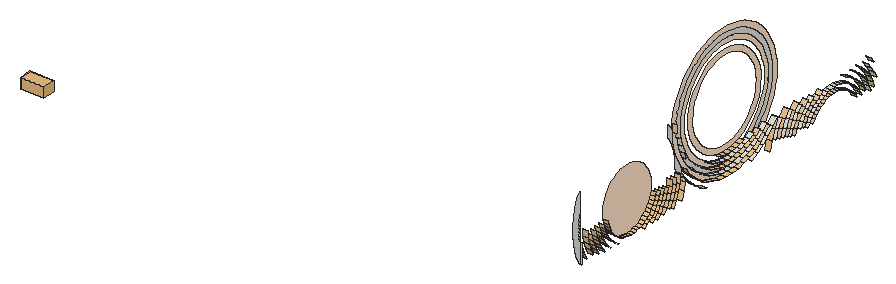
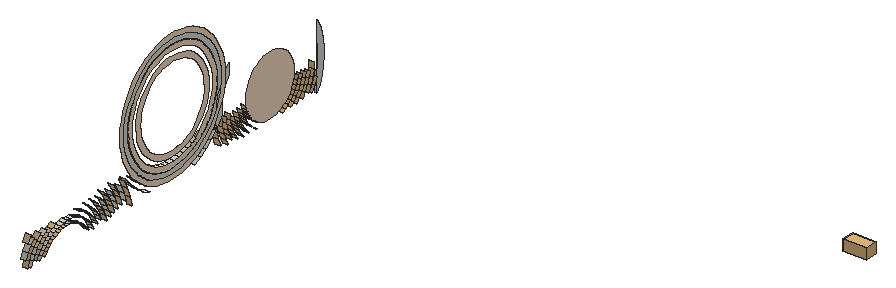
# SketchUp Ruby script. Lengths in inches.
U = 1.inch
M = Sketchup.active_model
def pt(a) = Geom::Point3d.new(a.map { |v| v * U })
def face(e, loops, mat)
  f = e.add_face(loops[0].map { |a| pt(a) })
  loops[1..].each { |l| e.add_face(l.map { |a| pt(a) }).erase! }
  f.material = f.back_material = mat if mat
  f
end
# faces: each face lists its corners as indices into pts; further lists are holes
def faces(e, pts, list, mat = nil) = list.each { |f| face(e, (f[0].is_a?(Array) ? f : [f]).map { |l| l.map { |i| pts[i] } }, mat) }
# xy, xz, yz: faces in a plane at the given z, y or x. An outline is a flat list of corners, or four numbers for a rectangle; further outlines are holes
def ring(l) = l.size == 4 ? [[l[0], l[1]], [l[2], l[1]], [l[2], l[3]], [l[0], l[3]]] : l.each_slice(2).to_a
def flat(e, list, mat, &to3) = list.each { |f| face(e, (f[0].is_a?(Array) ? f : [f]).map { |l| ring(l).map { |u, v| to3.(u, v) } }, mat) }
def xy(e, z, list, mat = nil) = flat(e, list, mat) { |x, y| [x, y, z] }
def xz(e, y, list, mat = nil) = flat(e, list, mat) { |x, z| [x, y, z] }
def yz(e, x, list, mat = nil) = flat(e, list, mat) { |y, z| [x, y, z] }
def lines(e, pts, list) = list.each { |a, b| e.add_line(pt(pts[a]), pt(pts[b])) }
# prism: a flat outline (further loops are holes) pulled along v
def prism(e, loops, v, mat = nil)
  f = face(e, loops, mat); d = Geom::Vector3d.new(v.map { |x| x * U })
  f.pushpull(f.normal.samedirection?(d) ? d.length : -d.length)
end
def box(e, o, s, mat = nil) = prism(e, [[o, [o[0] + s[0], o[1], o[2]], [o[0] + s[0], o[1] + s[1], o[2]], [o[0], o[1] + s[1], o[2]]]], [0, 0, s[2]], mat)
def at(x, y, z, deg = 0) = Geom::Transformation.translation(pt([x, y, z])) * Geom::Transformation.rotation(ORIGIN, Z_AXIS, deg.degrees)
def axes(o, x, y, z) = Geom::Transformation.new([*x, 0, *y, 0, *z, 0, *pt(o).to_a, 1])
def part(name) = M.definitions.add(name)
# library, detail: a bought-in or finely detailed component or shape, given as its bounding box
def library(name, o, s) = part(name).tap { |d| box(d.entities, o, s) }
def detail(e, o, s) = box(e.add_group.entities, o, s)
def put(e, d, t, mat = nil) = e.add_instance(d, t).tap { |i| i.material = mat if mat }
def group(e, t, mat = nil) = e.add_group.tap { |g| g.transformation = t; g.material = mat if mat }.entities
root = M.entities
M.materials.add("[Color C02]").color = [255, 228, 201]
M.materials.add("images").color = [235, 194, 141]
c1 = library("Group\#240",[-0.66,-0.65,0],[9.25,4.94,4.13])
xy(root,39.7,[[183.82,116.84,185.82,119.625]])
xy(root,41.7,[[183.82,116.96,185.82,119.51]],"images")
xz(root,46.5625,[[183.82,37.01,184.63,44.88]])
yz(root,183.82,[[46.5625,37.01,45.42,39.3125,44.37,42.24,43.67,45.27,43.32,48.36,43.34,51.47,43.71,54.56,44.44,57.58,45.52,60.49,46.5625,62.54,46.5625,54.71,46.41,54.07,46.07,51.3,46.05,48.51,46.36,45.73,46.5625,44.88],[[116.84,39.7,119.625,39.7,122.39,40.02,125.1,40.66,127.72,41.6,130.21,42.85,132.53,44.375,134.67,46.16,136.58,48.18,138.25,50.41,139.64,52.82,140.75,55.375,141.55,58.04,142.04,60.78,142.2,63.56,142.05,66.34,141.57,69.08,140.77,71.75,139.68,74.3,138.29,76.72,136.63,78.95,134.72,80.98,132.59,82.77,130.27,84.3,127.78,85.56,125.17,86.51,122.46,87.16,119.7,87.49,116.91,87.49,114.15,87.17,111.44,86.53,108.82,85.59,106.33,84.34,104.01,82.8125,101.87,81.03,99.96,79.01,98.29,76.78,96.9,74.37,95.79,71.8125,94.99,69.15,94.5,66.41,94.34,63.63,94.49,60.85,94.59,60.33,94.625,60.25,95.67,57.32,96.375,54.3,96.42,53.93,96.87,52.88,98.25,50.47,99.91,48.24,101.82,46.21,103.95,44.42,106.27,42.88,108.76,41.63,111.37,40.68,114.08,40.03],[116.96,41.7,114.43,42,111.95,42.59,109.55,43.47,107.27,44.62,105.15,46.02,103.19,47.66,101.45,49.52,99.93,51.57,98.65,53.78,97.65,56.125,96.92,58.57,96.48,61.08,96.34,63.63,96.49,66.17,96.94,68.68,97.67,71.13,98.68,73.47,99.96,75.67,101.49,77.72,103.24,79.57,105.2,81.21,107.33,82.61,109.61,83.75,112.01,84.62,114.49,85.2,117.03,85.49,119.58,85.49,122.11,85.19,124.59,84.6,126.99,83.72,129.27,82.57,131.4,81.17,133.35,79.53,135.09,77.67,136.61,75.62,137.89,73.41,138.89,71.07,139.62,68.62,140.06,66.11,140.2,63.5625,140.05,61.02,139.61,58.5,138.87,56.0625,137.86,53.72,136.58,51.51,135.05,49.47,133.3,47.62,131.34,45.98,129.21,44.58,126.93,43.44,124.53,42.57,122.05,41.99,119.51,41.7]],[[116.96,41.7,119.51,41.7,122.05,41.99,124.53,42.57,126.93,43.44,129.21,44.58,131.34,45.98,133.3,47.62,135.05,49.47,136.58,51.51,137.86,53.72,138.87,56.0625,139.61,58.5,140.05,61.02,140.2,63.5625,140.06,66.11,139.62,68.62,138.89,71.07,137.89,73.41,136.61,75.62,135.09,77.67,133.35,79.53,131.4,81.17,129.27,82.57,126.99,83.72,124.59,84.6,122.11,85.19,119.58,85.49,117.03,85.49,114.49,85.2,112.01,84.62,109.61,83.75,107.33,82.61,105.2,81.21,103.24,79.57,101.49,77.72,99.96,75.67,98.68,73.47,97.67,71.13,96.94,68.68,96.49,66.17,96.34,63.63,96.48,61.08,96.92,58.57,97.65,56.125,98.65,53.78,99.93,51.57,101.45,49.52,103.19,47.66,105.15,46.02,107.27,44.62,109.55,43.47,111.95,42.59,114.43,42],[116.96,41.71,114.43,42.01,111.95,42.6,109.56,43.48,107.28,44.625,105.15,46.03,103.2,47.67,101.45,49.53,99.94,51.57,98.66,53.78,97.66,56.125,96.93,58.57,96.49,61.08,96.35,63.63,96.5,66.17,96.94,68.68,97.68,71.125,98.69,73.46,99.97,75.67,101.5,77.71,103.25,79.5625,105.2,81.2,107.34,82.6,109.62,83.74,112.01,84.61,114.5,85.19,117.03,85.48,119.58,85.48,122.11,85.18,124.59,84.59,126.98,83.71,129.26,82.56,131.39,81.16,133.34,79.52,135.09,77.66,136.61,75.61,137.88,73.4,138.88,71.0625,139.61,68.62,140.05,66.11,140.19,63.5625,140.04,61.02,139.6,58.51,138.86,56.07,137.85,53.73,136.57,51.52,135.04,49.48,133.29,47.625,131.34,45.99,129.2,44.59,126.92,43.45,124.53,42.58,122.05,42,119.51,41.71]],[46.5625,44.88,46.36,45.73,46.05,48.51,46.07,51.3,46.41,54.07,46.5625,54.71],[96.47,46.17,96.71,48.1,96.71,49.2,96.58,49.375,95.08,51.99,93.89,54.76,93.03,57.65,92.51,60.62,92.34,63.63,92.38,64.36,91.55,65.64,90.53,66.87,90.34,63.64,90.41,62.38,90.86,61.68,92.1,59.18,93.05,56.55,93.68,53.83,93.99,51.06,93.98,49.89,94.91,48.28],
  [96.42,53.93,96.375,54.3,95.67,57.32,94.625,60.25,94.59,60.33,94.97,58.11,95.77,55.44]])
yz(root,183.82,[[[119.74,37.7,122.74,38.05,125.67,38.74,128.51,39.77,131.2,41.12,133.73,42.77,136.04,44.7,138.11,46.89,139.92,49.3125,141.43,51.92,142.63,54.6875,143.5,57.58,144.02,60.55,144.2,63.56,144.03,66.57,143.51,69.54,142.65,72.43,141.46,75.2,139.96,77.8125,138.16,80.23,136.1,82.43,133.79,84.375,131.27,86.03,128.58,87.39,125.75,88.43,122.8125,89.13,119.82,89.48,116.8,89.49,113.81,89.14,110.87,88.45,108.03,87.42,105.34,86.07,102.81,84.42,100.5,82.49,98.43,80.29,96.625,77.88,95.11,75.27,93.91,72.5,93.04,69.61,92.52,66.64,92.38,64.36,92.34,63.63,92.51,60.62,93.03,57.65,93.89,54.76,95.08,51.99,96.58,49.375,96.71,49.2,98.38,46.95,100.45,44.76,102.75,42.82,105.27,41.15,107.96,39.8,110.8,38.76,113.73,38.0625,116.72,37.71],[116.84,39.7,114.08,40.03,111.37,40.68,108.76,41.63,106.27,42.88,103.95,44.42,101.82,46.21,99.91,48.24,98.25,50.47,96.87,52.88,96.42,53.93,95.77,55.44,94.97,58.11,94.59,60.33,94.49,60.85,94.34,63.63,94.5,66.41,94.99,69.15,95.79,71.8125,96.9,74.37,98.29,76.78,99.96,79.01,101.87,81.03,104.01,82.8125,106.33,84.34,108.82,85.59,111.44,86.53,114.15,87.17,116.91,87.49,119.7,87.49,122.46,87.16,125.17,86.51,127.78,85.56,130.27,84.3,132.59,82.77,134.72,80.98,136.63,78.95,138.29,76.72,139.68,74.3,140.77,71.75,141.57,69.08,142.05,66.34,142.2,63.56,142.04,60.78,141.55,58.04,140.75,55.375,139.64,52.82,138.25,50.41,136.58,48.18,134.67,46.16,132.53,44.375,130.21,42.85,127.72,41.6,125.1,40.66,122.39,40.02,119.625,39.7]],[69.96,37.78,71.35,37.86,72.73,38.09,74.07,38.49,75.35,39.03,76.57,39.72,77.6875,40.55,78.71,41.51,79.61,42.57,80.38,43.73,81.02,44.98,81.5,46.28,81.83,47.64,82,49.03,82,50.42,81.85,51.81,81.53,53.17,81.0625,54.48,80.44,55.73,79.68,56.9,78.79,57.97,77.78,58.9375,76.66,59.78,75.46,60.48,74.18,61.04,72.85,61.45,71.47,61.69,70.08,61.78,68.6875,61.71,67.3125,61.47,65.97,61.08,64.6875,60.53,63.48,59.84,62.35,59.01,61.33,58.0625,60.43,57,59.66,55.83,59.03,54.59,58.54,53.28,58.21,51.93,58.04,50.54,58.04,49.14,58.19,47.76,58.51,46.4,58.98,45.08,59.6,43.83,60.36,42.66,61.25,41.59,62.26,40.63,63.38,39.79,64.58,39.09,65.86,38.53,67.2,38.12,68.57,37.87],[[116.96,41.71,119.51,41.71,122.05,42,124.53,42.58,126.92,43.45,129.2,44.59,131.34,45.99,133.29,47.625,135.04,49.48,136.57,51.52,137.85,53.73,138.86,56.07,139.6,58.51,140.04,61.02,140.19,63.5625,140.05,66.11,139.61,68.62,138.88,71.0625,137.88,73.4,136.61,75.61,135.09,77.66,133.34,79.52,131.39,81.16,129.26,82.56,126.98,83.71,124.59,84.59,122.11,85.18,119.58,85.48,117.03,85.48,114.5,85.19,112.01,84.61,109.62,83.74,107.34,82.6,105.2,81.2,103.25,79.5625,101.5,77.71,99.97,75.67,98.69,73.46,97.68,71.125,96.94,68.68,96.5,66.17,96.35,63.63,96.49,61.08,96.93,58.57,97.66,56.125,98.66,53.78,99.94,51.57,101.45,49.53,103.2,47.67,105.15,46.03,107.28,44.625,109.56,43.48,111.95,42.6,114.43,42.01],[119.4,43.69,117.08,43.7,114.78,43.97,112.52,44.51,110.35,45.3,108.28,46.35,106.34,47.62,104.57,49.12,102.98,50.8,101.6,52.67,100.44,54.67,99.53,56.8,98.87,59.03,98.47,61.31,98.34,63.625,98.47,65.9375,98.88,68.22,99.55,70.44,100.47,72.57,101.63,74.57,103.02,76.43,104.61,78.11,106.39,79.6,108.33,80.87,110.4,81.91,112.58,82.7,114.84,83.23,117.14,83.5,119.46,83.49,121.76,83.22,124.02,82.68,126.19,81.89,128.26,80.84,130.2,79.57,131.97,78.07,133.56,76.39,134.94,74.52,136.1,72.51,137.01,70.38,137.67,68.16,138.07,65.88,138.2,63.56,138.07,61.25,137.66,58.97,136.99,56.75,136.07,54.62,134.91,52.62,133.52,50.76,131.93,49.07,130.15,47.59,128.21,46.32,126.14,45.28,123.96,44.49,121.7,43.96]],[[119.29,45.6875,121.36,45.93,123.39,46.41,125.35,47.12,127.21,48.05,128.96,49.19,130.56,50.53,131.99,52.05,133.24,53.72,134.29,55.52,135.11,57.44,135.72,59.43,136.08,61.49,136.2,63.57,136.09,65.65,135.73,67.7,135.13,69.7,134.31,71.62,133.27,73.43,132.03,75.1,130.6,76.62,129,77.96,127.26,79.11,125.4,80.05,123.44,80.77,121.41,81.25,119.34,81.5,117.25,81.5,115.18,81.26,113.15,80.78,111.19,80.07,109.33,79.14,107.58,78,105.98,76.66,104.55,75.14,103.3,73.47,102.26,71.67,101.43,69.75,100.83,67.76,100.46,65.7,100.34,63.62,100.45,61.54,100.8125,59.48,101.41,57.49,102.23,55.57,103.27,53.76,104.51,52.09,105.94,50.57,107.54,49.23,109.28,48.08,111.14,47.14,113.1,46.42,115.13,45.9375,117.2,45.69],[117.32,47.6875,115.48,47.91,113.68,48.34,111.9375,48.97,110.28,49.81,108.74,50.83,107.32,52.02,106.05,53.37,104.94,54.86,104.02,56.46,103.29,58.17,102.76,59.94,102.44,61.77,102.34,63.62,102.45,65.47,102.77,67.29,103.31,69.07,104.04,70.77,104.97,72.37,106.08,73.86,107.35,75.2,108.77,76.39,110.32,77.41,111.98,78.24,113.72,78.87,115.53,79.29,117.37,79.5,119.22,79.5,121.0625,79.28,122.86,78.85,124.6,78.22,126.26,77.38,127.81,76.36,129.22,75.17,130.49,73.82,131.6,72.33,132.52,70.72,133.25,69.02,133.78,67.25,134.1,65.42,134.2,63.57,134.09,61.72,133.77,59.9,133.24,58.12,132.5,56.42,131.57,54.82,130.46,53.33,129.1875,51.99,127.77,50.8,126.22,49.78,124.56,48.95,122.82,48.32,121.01,47.9,119.17,47.6875]]],"[Color C02]")
p = [[183.82,139.31,40.71],[183.82,138.46,37.03],[185.82,138.46,37.03],[185.82,139.31,40.71],[183.82,187.32,38.99],[183.82,188.07,36.98],
  [185.82,188.07,36.98],[185.82,187.32,38.99],[183.82,76.24,37.24],[183.82,77.66,38.05],[185.82,77.66,38.05],[185.82,76.24,37.24],
  [183.82,157.14,37.23],[183.82,157.89,38.73],[185.82,157.89,38.73],[185.82,157.14,37.23],[183.82,62.27,38.125],[183.82,63.68,37.3],
  [185.82,63.68,37.3],[185.82,62.27,38.125],[183.82,151.62,39.57],[183.82,150.82,37.34],[185.82,150.82,37.34],[185.82,151.62,39.57],
  [183.82,83.05,37.37],[183.82,84.41,38.96],[185.82,84.41,38.96],[185.82,83.05,37.37],[183.82,182.89,38.88],[183.82,183.66,37.39],
  [185.82,183.66,37.39],[185.82,182.89,38.88],[183.82,55.53,39.11],[183.82,56.87,37.5],[185.82,56.87,37.5],[185.82,55.53,39.11],
  [183.82,81.6,38.75],[183.82,80.24,37.48],[185.82,80.24,37.48],[185.82,81.6,38.75],[183.82,59.68,37.58],[183.82,58.33,38.86],
  [185.82,58.33,38.86],[185.82,59.68,37.58],[183.82,189.98,37.57],[183.82,189.15,39.79],[185.82,189.15,39.79],[185.82,189.98,37.57],
  [183.82,92.01,40.17],[183.82,90.75,37.68],[185.82,90.75,37.68],[185.82,92.01,40.17],[183.82,116.72,37.71],[183.82,113.73,38.0625],
  [185.82,113.73,38.0625],[185.82,116.72,37.71],[183.82,119.74,37.7],[185.82,119.74,37.7],[183.82,122.74,38.05],[185.82,122.74,38.05],
  [183.82,160.41,38.96],[183.82,159.625,37.74],[185.82,159.625,37.74],[185.82,160.41,38.96],[183.82,69.96,37.78],[183.82,68.57,37.87],
  [185.82,68.57,37.87],[185.82,69.96,37.78],[183.82,71.35,37.86],[185.82,71.35,37.86],[183.82,87.29,39.7],[183.82,86,37.76],
  [185.82,86,37.76],[185.82,87.29,39.7],[183.82,49.18,37.89],[183.82,47.9375,40.39],[184.63,47.9375,40.39],[184.63,49.18,37.89],
  [183.82,53.92,37.92],[183.82,52.65,39.87],[185.82,52.65,39.87],[185.82,53.92,37.92],[183.82,67.2,38.12],[185.82,67.2,38.12],
  [183.82,72.73,38.09],[185.82,72.73,38.09],[183.82,129.3,37.93],[183.82,132.2,39.38],[185.82,132.2,39.38],[185.82,129.3,37.93],
  [183.82,148.9,37.9],[183.82,149.78,40.35],[185.82,149.78,40.35],[185.82,148.9,37.9],[183.82,181.17,37.87],[183.82,180.37,39.08],
  [185.82,180.37,39.08],[185.82,181.17,37.87],[183.82,78.97,39.01],[185.82,78.97,39.01],[183.82,104.27,39.42],[183.82,107.17,37.96],
  [185.82,107.17,37.96],[185.82,104.27,39.42],[183.82,125.67,38.74],[185.82,125.67,38.74],[183.82,156.15,39.72],[183.82,155.3,38.01],
  [185.82,155.3,38.01],[185.82,156.15,39.72],[183.82,60.97,39.1],[185.82,60.97,39.1],[183.82,65.86,38.53],[185.82,65.86,38.53],
  [183.82,74.07,38.49],[185.82,74.07,38.49],[183.82,110.8,38.76],[185.82,110.8,38.76],[183.82,185.49,38.1875],[183.82,184.62,39.89],
  [185.82,184.62,39.89],[185.82,185.49,38.1875],[183.82,64.58,39.09],[185.82,64.58,39.09],[183.82,75.35,39.03],[185.82,75.35,39.03],
  [183.82,147.9375,41.14],[183.82,146.98,38.46],[185.82,146.98,38.46],[185.82,147.9375,41.14],[183.82,82.81,40.17],[185.82,82.81,40.17],
  [183.82,89.02,38.6875],[183.82,90.18,40.97],[185.82,90.18,40.97],[185.82,89.02,38.6875],[183.82,128.51,39.77],[185.82,128.51,39.77],
  [183.82,158.8,40.14],[185.82,158.8,40.14],[183.82,107.96,39.8],[185.82,107.96,39.8],[183.82,153.46,38.79],[183.82,154.41,40.71],
  [185.82,154.41,40.71],[185.82,153.46,38.79],[183.82,49.78,41.17],[183.82,50.91,38.88],[185.82,50.91,38.88],[185.82,49.78,41.17],
  [183.82,57.14,40.29],[185.82,57.14,40.29],[183.82,181.96,40.28],[185.82,181.96,40.28],[183.82,76.57,39.72],[185.82,76.57,39.72],
  [183.82,80.16,40.125],[185.82,80.16,40.125],[183.82,85.5625,40.71],[185.82,85.5625,40.71],[183.82,145.0625,39.02],[183.82,146.1,41.92],
  [185.82,146.1,41.92],[185.82,145.0625,39.02],[183.82,161.34,40.07],[185.82,161.34,40.07],[183.82,186.35,40.9],[185.82,186.35,40.9],
  [183.82,54.39,40.86],[185.82,54.39,40.86],[183.82,59.79,40.23],[185.82,59.79,40.23],[183.82,63.38,39.79],[185.82,63.38,39.79],
  [183.82,94.52,39.07],[183.82,95.6,41.99],[185.82,95.6,41.99],[185.82,94.52,39.07],[183.82,179.43,40.18],[185.82,179.43,40.18],
  [183.82,101.56,41.21],[185.82,101.56,41.21],[183.82,134.92,41.16],[185.82,134.92,41.16],[183.82,144.26,42.7],[183.82,143.14,39.58],
  [185.82,143.14,39.58],[185.82,144.26,42.7],[183.82,152.67,41.7],[185.82,152.67,41.7],[183.82,77.6875,40.55],[185.82,77.6875,40.55],
  [183.82,88.35,41.77],[185.82,88.35,41.77],[183.82,114.08,40.03],[183.82,116.84,39.7],[185.82,116.84,39.7],[185.82,114.08,40.03],
  [183.82,119.625,39.7],[183.82,122.39,40.02],[185.82,122.39,40.02],[185.82,119.625,39.7],[183.82,157.19,41.33],[185.82,157.19,41.33],
  [183.82,62.26,40.63],[185.82,62.26,40.63],[183.82,105.27,41.15],[185.82,105.27,41.15],[183.82,131.2,41.12],[185.82,131.2,41.12],
  [183.82,188.07,41.91],[185.82,188.07,41.91],[183.82,51.62,41.95],[185.82,51.62,41.95],[183.82,183.5625,41.48],[185.82,183.5625,41.48],
  [183.82,111.37,40.68],[185.82,111.37,40.68],[183.82,125.1,40.66],[185.82,125.1,40.66],[183.82,81.21,41.37],[185.82,81.21,41.37],
  [183.82,141.22,40.15],[183.82,142.42,43.48],[185.82,142.42,43.48],[185.82,141.22,40.15],[183.82,159.875,41.43],[185.82,159.875,41.43],
  [183.82,162.38,41.07],[185.82,162.38,41.07],[183.82,58.75,41.48],[185.82,58.75,41.48],[183.82,83.84,41.71],[185.82,83.84,41.71],
  [183.82,92.98,42.79],[185.82,92.98,42.79],[183.82,178.37,41.16],[185.82,178.37,41.16],[183.82,56.125,41.85],[185.82,56.125,41.85],
  [183.82,180.88,41.56],[185.82,180.88,41.56],[183.82,47,43.01],[184.63,47,43.01],[183.82,150.9375,42.69],[185.82,150.9375,42.69],
  [183.82,61.25,41.59],[185.82,61.25,41.59],[183.82,78.71,41.51],[185.82,78.71,41.51],[183.82,189.8,42.92],[183.82,190.98,40.6],
  [185.82,190.98,40.6],[185.82,189.8,42.92],[183.82,86.51,42.57],[185.82,86.51,42.57],[183.82,108.76,41.63],[185.82,108.76,41.63],
  [183.82,127.72,41.6],[185.82,127.72,41.6],[183.82,140.57,44.26],[185.82,140.57,44.26],[183.82,155.58,42.51],[185.82,155.58,42.51],
  [183.82,53.46,42.74],[185.82,53.46,42.74],[183.82,185.16,42.6875],[185.82,185.16,42.6875],[183.82,91.06,43.37],[185.82,91.06,43.37],
  [183.82,133.73,42.77],[185.82,133.73,42.77],[183.82,149.2,43.68],[185.82,149.2,43.68],[183.82,163.54,41.94],[185.82,163.54,41.94],
  [183.82,48.91,43.58],[185.82,48.91,43.58],[183.82,99.07,43.3],[185.82,99.07,43.3],[183.82,102.75,42.82],[185.82,102.75,42.82],
  [183.82,137.41,43.25],[185.82,137.41,43.25],[183.82,177.21,42.02],[185.82,177.21,42.02],[183.82,158.41,42.8],[185.82,158.41,42.8],
  [183.82,82.11,42.72],[185.82,82.11,42.72],[183.82,161.09,42.59],[185.82,161.09,42.59],[183.82,57.86,42.84],[185.82,57.86,42.84],
  [183.82,79.61,42.57],[185.82,79.61,42.57],[183.82,182.32,42.94],[185.82,182.32,42.94],[183.82,60.36,42.66],[185.82,60.36,42.66],
  [183.82,106.27,42.88],[185.82,106.27,42.88],[183.82,130.21,42.85],[185.82,130.21,42.85],[183.82,179.65,42.7],[185.82,179.65,42.7],
  [183.82,84.68,43.375],[185.82,84.68,43.375],[183.82,116.96,41.7],[183.82,114.43,42],[185.82,114.43,42],[185.82,116.96,41.7],
  [183.82,122.05,41.99],[183.82,119.51,41.7],[185.82,119.51,41.7],[185.82,122.05,41.99],[183.82,153.97,43.7],[185.82,153.97,43.7],
  [183.82,89.15,43.95],[185.82,89.15,43.95],[183.82,55.3,43.52],[185.82,55.3,43.52],[183.82,147.46,44.67],[185.82,147.46,44.67],
  [183.82,164.79,42.67],[185.82,164.79,42.67],[183.82,186.76,43.89],[185.82,186.76,43.89],[183.82,50.83,44.14],[185.82,50.83,44.14],
  [183.82,96.33,45.01],[185.82,96.33,45.01],[183.82,111.95,42.59],[185.82,111.95,42.59],[183.82,124.53,42.57],[185.82,124.53,42.57],
  [183.82,175.95,42.74],[185.82,175.95,42.74],[183.82,156.95,44.16],[185.82,156.95,44.16],[183.82,80.38,43.73],[185.82,80.38,43.73],
  [183.82,87.24,44.54],[185.82,87.24,44.54],[183.82,109.55,43.47],[185.82,109.55,43.47],[183.82,126.93,43.44],[185.82,126.93,43.44],
  [183.82,162.43,43.6],[185.82,162.43,43.6],[183.82,52.75,44.71],[185.82,52.75,44.71],[183.82,59.6,43.83],[185.82,59.6,43.83],
  [183.82,82.85,44.17],[185.82,82.85,44.17],[183.82,145.72,45.66],[185.82,145.72,45.66],[183.82,152.36,44.88],[185.82,152.36,44.88],
  [183.82,166.11,43.25],[185.82,166.11,43.25],[183.82,174.62,43.3],[185.82,174.62,43.3],[183.82,178.3,43.7],[185.82,178.3,43.7],
  [183.82,183.77,44.32],[185.82,183.77,44.32],[183.82,57.14,44.3],[185.82,57.14,44.3],[183.82,93.64,45.5],[185.82,93.64,45.5],
  [183.82,100.45,44.76],[185.82,100.45,44.76],[183.82,132.53,44.375],[185.82,132.53,44.375],[183.82,136.04,44.7],[185.82,136.04,44.7],
  [183.82,159.79,44.12],[185.82,159.79,44.12],[183.82,103.95,44.42],[185.82,103.95,44.42],[183.82,180.93,44.24],[185.82,180.93,44.24],
  [183.82,188.35,45.09],[185.82,188.35,45.09],[183.82,46.5625,44.88],[184.63,46.5625,44.88],[183.82,139.64,45.61],[185.82,139.64,45.61],
  [183.82,96.84,45.67],[185.82,96.84,45.67],[183.82,167.49,43.67],[185.82,167.49,43.67],[183.82,173.23,43.71],[185.82,173.23,43.71],
  [183.82,85.33,45.12],[185.82,85.33,45.12],[183.82,91.67,45.86],[185.82,91.67,45.86],[183.82,129.21,44.58],[185.82,129.21,44.58],
  [183.82,54.67,45.27],[185.82,54.67,45.27],[183.82,107.27,44.62],[185.82,107.27,44.62],[183.82,143.99,46.65],[185.82,143.99,46.65],
  [183.82,48.34,46.07],[185.82,48.34,46.07],[183.82,163.88,44.45],[185.82,163.88,44.45],[183.82,81.02,44.98],[185.82,81.02,44.98],
  [183.82,114.78,43.97],[183.82,117.08,43.7],[185.82,117.08,43.7],[185.82,114.78,43.97],[183.82,119.4,43.69],[185.82,119.4,43.69],
  [183.82,121.7,43.96],[185.82,121.7,43.96],[183.82,150.75,46.07],[185.82,150.75,46.07],[183.82,155.49,45.53],[185.82,155.49,45.53],
  [183.82,168.92,43.93],[185.82,168.92,43.93],[183.82,171.81,43.95],[185.82,171.81,43.95],[183.82,176.84,44.53],[185.82,176.84,44.53],
  [183.82,58.98,45.08],[185.82,58.98,45.08],[183.82,170.36,44.03],[185.82,170.36,44.03],[183.82,185.22,45.7],[185.82,185.22,45.7],
  [183.82,89.7,46.21],[185.82,89.7,46.21],[183.82,112.52,44.51],[185.82,112.52,44.51],[183.82,123.96,44.49],[185.82,123.96,44.49],
  [183.82,50.31,46.41],[185.82,50.31,46.41],[183.82,161.32,45.27],[185.82,161.32,45.27],[183.82,83.41,45.7],[185.82,83.41,45.7],
  [183.82,158.5,45.64],[185.82,158.5,45.64],[183.82,179.39,45.375],[185.82,179.39,45.375],[183.82,56.59,45.83],[185.82,56.59,45.83],
  [183.82,142.25,47.64],[185.82,142.25,47.64],[183.82,182.2,45.78],[185.82,182.2,45.78],[183.82,101.82,46.21],[185.82,101.82,46.21],
  [183.82,134.67,46.16],[185.82,134.67,46.16],[183.82,87.73,46.57],[185.82,87.73,46.57],[183.82,110.35,45.3],[185.82,110.35,45.3],
  [183.82,126.14,45.28],[185.82,126.14,45.28],[183.82,165.42,45.125],[185.82,165.42,45.125],[183.82,175.29,45.18],[185.82,175.29,45.18],
  [183.82,105.15,46.02],[185.82,105.15,46.02],[183.82,131.34,45.98],[185.82,131.34,45.98],[183.82,52.28,46.75],[185.82,52.28,46.75],
  [183.82,138.11,46.89],[185.82,138.11,46.89],[183.82,149.14,47.25],[185.82,149.14,47.25],[183.82,98.38,46.95],[185.82,98.38,46.95],
  [183.82,154.02,46.89],[185.82,154.02,46.89],[183.82,81.5,46.28],[185.82,81.5,46.28],[183.82,96.47,46.17],[185.82,96.47,46.17],
  [183.82,58.51,46.4],[185.82,58.51,46.4],[183.82,85.76,46.93],[185.82,85.76,46.93],[183.82,167.02,45.62],[185.82,167.02,45.62],
  [183.82,186.66,47.08],[185.82,186.66,47.08],[183.82,173.68,45.66],[185.82,173.68,45.66],[183.82,54.25,47.08],[185.82,54.25,47.08],
  [183.82,108.28,46.35],[185.82,108.28,46.35],[183.82,128.21,46.32],[185.82,128.21,46.32],[183.82,162.97,46.23],[185.82,162.97,46.23],
  [183.82,177.72,46.32],[185.82,177.72,46.32],[183.82,93.97,48.27],[185.82,93.97,48.27],[183.82,157.21,47.17],[185.82,157.21,47.17],
  [183.82,141.59,48.21],[185.82,141.59,48.21],[183.82,160.21,46.93],[185.82,160.21,46.93],[183.82,168.67,45.92],[185.82,168.67,45.92],
  [183.82,83.8,47.28],[185.82,83.8,47.28],[183.82,117.2,45.69],[183.82,115.13,45.9375],[185.82,115.13,45.9375],[185.82,117.2,45.69],
  [183.82,119.29,45.6875],[185.82,119.29,45.6875],[183.82,121.36,45.93],[185.82,121.36,45.93],[183.82,147.52,48.4375],[185.82,147.52,48.4375],
  [183.82,172.03,45.9375],[185.82,172.03,45.9375],[183.82,183.48,47.32],[185.82,183.48,47.32],[183.82,56.22,47.42],[185.82,56.22,47.42],
  [183.82,180.47,47.05],[185.82,180.47,47.05],[183.82,91.98,48.4],[185.82,91.98,48.4],[183.82,113.1,46.42],[185.82,113.1,46.42],
  [183.82,123.39,46.41],[185.82,123.39,46.41],[183.82,170.35,46.03],[185.82,170.35,46.03],[183.82,103.19,47.66],[185.82,103.19,47.66],
  [183.82,133.3,47.62],[185.82,133.3,47.62],[183.82,48.05,48.61],[185.82,48.05,48.61],[183.82,152.56,48.25],[185.82,152.56,48.25],
  [183.82,89.98,48.52],[185.82,89.98,48.52],[183.82,94.91,48.28],[185.82,94.91,48.28],[183.82,99.91,48.24],[185.82,99.91,48.24],
  [183.82,136.58,48.18],[185.82,136.58,48.18],[183.82,164.72,47],[185.82,164.72,47],[183.82,81.83,47.64],[185.82,81.83,47.64],
  [183.82,106.34,47.62],[185.82,106.34,47.62],[183.82,130.15,47.59],[185.82,130.15,47.59],[183.82,175.96,47.07],[185.82,175.96,47.07],
  [183.82,189.95,46.3],[183.82,188.11,48.46],[185.82,188.11,48.46],[185.82,189.95,46.3],[183.82,58.19,47.76],[185.82,58.19,47.76],
  [183.82,125.35,47.12],[185.82,125.35,47.12],[183.82,96.71,49.2],[183.82,96.58,49.375],[185.82,96.58,49.375],[183.82,96.42,53.93],
  [183.82,96.87,52.88],[185.82,96.87,52.88],[185.82,95.77,55.44],[183.82,95.77,55.44],[183.82,94.59,60.33],[183.82,94.97,58.11],
  [185.82,94.97,58.11],[185.82,94.49,60.85],[183.82,94.49,60.85],[183.82,92.34,63.63],[183.82,92.38,64.36],[183.82,92.52,66.64],
  [185.82,92.52,66.64],[185.82,92.34,63.63]]
faces(root,p,[[0,1,2,3],[8,9,10,11],[16,17,18,19],[20,21,22,23],[24,25,26,27],[32,33,34,35],[36,37,38,39],[40,41,42,43],
  [44,45,46,47],[48,49,50,51],[52,53,54,55],[56,52,55,57],[58,56,57,59],[60,61,62,63],[64,65,66,67],[68,64,67,69],
  [70,71,72,73],[74,75,76,77],[78,79,80,81],[65,82,83,66],[84,68,69,85],[94,95,96,97],[9,98,99,10],[104,58,59,105],
  [106,107,108,109],[110,16,19,111],[82,112,113,83],[114,84,85,115],[53,116,117,54],[118,119,120,121],[112,122,123,113],[124,114,115,125],
  [126,127,128,129],[130,36,39,131],[132,133,134,135],[136,104,105,137],[116,140,141,117],[146,147,148,149],[41,150,151,42],[154,124,125,155],
  [98,156,157,99],[25,158,159,26],[164,60,63,165],[168,32,35,169],[170,110,111,171],[122,172,173,123],[174,175,176,177],[95,178,179,96],
  [184,185,186,187],[188,20,23,189],[190,154,155,191],[192,70,73,193],[202,106,109,203],[172,204,205,173],[140,206,207,141],[208,136,137,209],
  [45,210,211,46],[79,212,213,80],[119,214,215,120],[156,220,221,157],[228,164,165,229],[230,170,171,231],[232,130,131,233],[234,48,51,235],
  [178,236,237,179],[150,238,239,151],[75,242,243,76],[204,246,247,205],[248,190,191,249],[158,254,255,159],[260,0,3,261],[264,168,169,265],
  [133,268,269,134],[270,208,209,271],[272,126,129,273],[274,228,229,275],[276,146,149,277],[206,280,281,207],[236,284,285,237],[286,202,203,287],
  [220,288,289,221],[292,230,231,293],[294,248,249,295],[214,296,297,215],[246,298,299,247],[306,232,233,307],[308,309,310,311],[312,313,314,315],
  [316,188,189,317],[318,192,193,319],[238,320,321,239],[324,274,275,325],[210,326,327,211],[212,328,329,213],[175,330,331,176],[309,332,333,310],
  [334,312,315,335],[284,336,337,285],[340,294,295,341],[254,342,343,255],[332,344,345,333],[346,334,335,347],[350,264,265,351],[298,352,353,299],
  [288,354,355,289],[356,184,187,357],[360,324,325,361],[336,362,363,337],[368,292,293,369],[370,234,235,371],[280,372,373,281],[376,270,271,377],
  [378,286,287,379],[296,382,383,297],[242,386,387,243],[392,360,361,393],[362,394,395,363],[396,306,307,397],[268,398,399,269],[400,346,347,401],
  [320,402,403,321],[344,404,405,345],[408,276,277,409],[412,340,341,413],[422,272,273,423],[424,316,317,425],[426,392,393,427],[394,428,429,395],
  [352,432,433,353],[434,426,427,435],[326,436,437,327],[438,318,319,439],[428,434,435,429],[328,444,445,329],[446,378,379,447],[354,448,449,355],
  [382,452,453,383],[454,368,369,455],[456,260,261,457],[342,464,465,343],[404,474,475,405],[476,400,401,477],[478,350,351,479],[480,376,377,481],
  [372,484,485,373],[488,412,413,489],[330,490,491,331],[432,492,493,433],[494,396,397,495],[402,502,503,403],[508,446,447,509],[452,510,511,453],
  [512,370,371,513],[514,424,425,515],[448,522,523,449],[524,525,526,527],[528,524,527,529],[530,528,529,531],[532,356,357,533],[436,536,537,437],
  [538,454,455,539],[398,542,543,399],[525,544,545,526],[546,530,531,547],[474,550,551,475],[552,476,477,553],[554,408,409,555],[556,422,423,557],
  [558,438,439,559],[566,508,509,567],[568,488,489,569],[510,574,575,511],[576,577,578,579],[492,580,581,493],[582,546,547,583],[484,584,585,586,485],
  [597,598,599,600,601]],"images")
faces(root,p,[[4,5,6,7],[12,13,14,15],[28,29,30,31],[86,87,88,89],[90,91,92,93],[100,101,102,103],[13,138,139,14],[142,143,144,145],
  [152,28,31,153],[160,161,162,163],[166,4,7,167],[180,100,103,181],[87,182,183,88],[194,195,196,197],[198,199,200,201],[216,194,197,217],
  [199,218,219,200],[222,223,224,225],[138,226,227,139],[240,152,153,241],[91,244,245,92],[250,251,252,253],[256,216,217,257],[218,258,259,219],
  [143,262,263,144],[266,166,167,267],[278,180,181,279],[182,282,283,183],[226,290,291,227],[300,256,257,301],[258,302,303,259],[304,240,241,305],
  [161,322,323,162],[262,338,339,263],[290,348,349,291],[244,358,359,245],[364,304,305,365],[366,266,267,367],[302,374,375,303],[380,300,301,381],
  [384,250,253,385],[282,388,389,283],[390,278,279,391],[223,406,407,224],[348,410,411,349],[414,415,416,417],[415,418,419,416],[418,420,421,419],
  [430,364,365,431],[440,414,417,441],[420,442,443,421],[338,450,451,339],[458,366,367,459],[460,380,381,461],[374,462,463,375],[466,440,441,467],
  [442,468,469,443],[410,470,471,411],[472,430,431,473],[322,482,483,323],[358,486,487,359],[470,496,497,471],[498,384,385,499],[500,472,473,501],
  [504,466,467,505],[468,506,507,469],[388,516,517,389],[450,518,519,451],[496,520,521,497],[490,390,391,491],[534,500,501,535],[540,458,459,541],
  [520,548,549,521],[548,534,535,549],[560,490,491,561],[562,460,461,563],[462,564,565,463],[570,504,505,571],[506,572,573,507],[587,588,589,590,591],
  [592,593,594,595,596]])
put(root,c1,at(-16.66,22.05,39.37))
